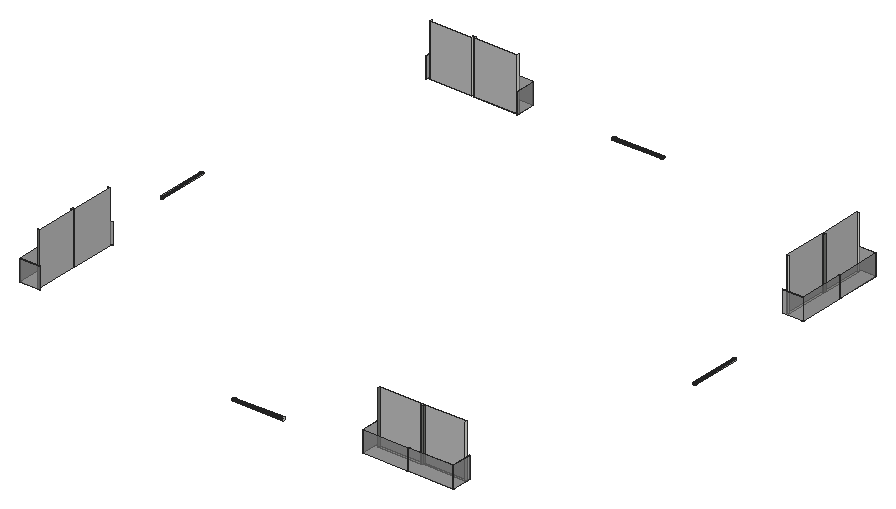
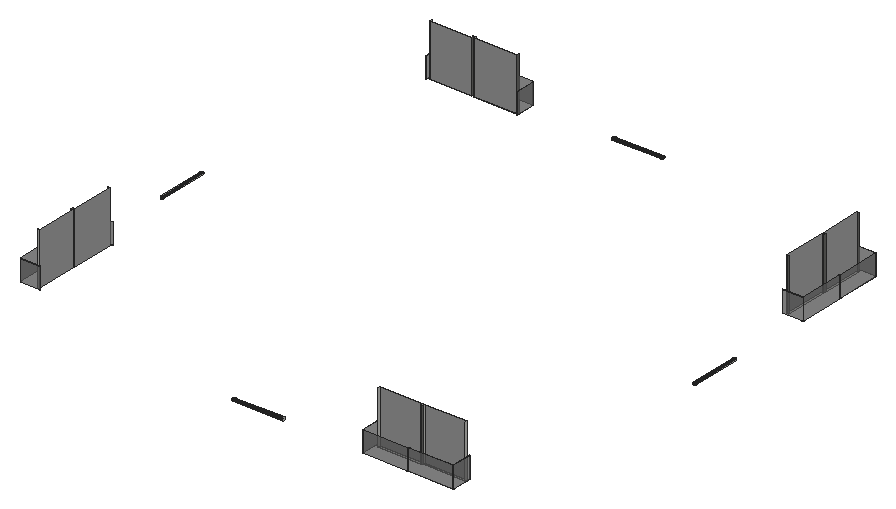
# SketchUp Ruby script. Lengths in inches.
U = 1.inch
M = Sketchup.active_model
def pt(a) = Geom::Point3d.new(a.map { |v| v * U })
def face(e, loops, mat)
  f = e.add_face(loops[0].map { |a| pt(a) })
  loops[1..].each { |l| e.add_face(l.map { |a| pt(a) }).erase! }
  f.material = f.back_material = mat if mat
  f
end
# faces: each face lists its corners as indices into pts; further lists are holes
def faces(e, pts, list, mat = nil) = list.each { |f| face(e, (f[0].is_a?(Array) ? f : [f]).map { |l| l.map { |i| pts[i] } }, mat) }
# xy, xz, yz: faces in a plane at the given z, y or x. An outline is a flat list of corners, or four numbers for a rectangle; further outlines are holes
def ring(l) = l.size == 4 ? [[l[0], l[1]], [l[2], l[1]], [l[2], l[3]], [l[0], l[3]]] : l.each_slice(2).to_a
def flat(e, list, mat, &to3) = list.each { |f| face(e, (f[0].is_a?(Array) ? f : [f]).map { |l| ring(l).map { |u, v| to3.(u, v) } }, mat) }
def xy(e, z, list, mat = nil) = flat(e, list, mat) { |x, y| [x, y, z] }
def xz(e, y, list, mat = nil) = flat(e, list, mat) { |x, z| [x, y, z] }
def yz(e, x, list, mat = nil) = flat(e, list, mat) { |y, z| [x, y, z] }
def lines(e, pts, list) = list.each { |a, b| e.add_line(pt(pts[a]), pt(pts[b])) }
# prism: a flat outline (further loops are holes) pulled along v
def prism(e, loops, v, mat = nil)
  f = face(e, loops, mat); d = Geom::Vector3d.new(v.map { |x| x * U })
  f.pushpull(f.normal.samedirection?(d) ? d.length : -d.length)
end
def box(e, o, s, mat = nil) = prism(e, [[o, [o[0] + s[0], o[1], o[2]], [o[0] + s[0], o[1] + s[1], o[2]], [o[0], o[1] + s[1], o[2]]]], [0, 0, s[2]], mat)
def at(x, y, z, deg = 0) = Geom::Transformation.translation(pt([x, y, z])) * Geom::Transformation.rotation(ORIGIN, Z_AXIS, deg.degrees)
def axes(o, x, y, z) = Geom::Transformation.new([*x, 0, *y, 0, *z, 0, *pt(o).to_a, 1])
def part(name) = M.definitions.add(name)
# library, detail: a bought-in or finely detailed component or shape, given as its bounding box
def library(name, o, s) = part(name).tap { |d| box(d.entities, o, s) }
def detail(e, o, s) = box(e.add_group.entities, o, s)
def put(e, d, t, mat = nil) = e.add_instance(d, t).tap { |i| i.material = mat if mat }
def group(e, t, mat = nil) = e.add_group.tap { |g| g.transformation = t; g.material = mat if mat }.entities
root = M.entities
M.materials.add("[Metal Seamed]").color = [118, 119, 115]
M.materials.add("[Mirror 01]").color = [185, 185, 185]
M.materials.add("[Translucent Glass Tinted]").color = [8, 201, 241]
M.materials["[Translucent Glass Tinted]"].alpha = 0.48
M.materials.add("[Translucent_Glass_Gray]").color = [128, 128, 128]
M.materials["[Translucent_Glass_Gray]"].alpha = 0.5
c1 = part("gler")
box(c1.entities,[0,-0.71,0],[0.37,57.8,41.34],"[Translucent_Glass_Gray]")
xy(root,1219.11,[[1161.2,84.8125,1285.04,90.8125],[1291.04,84.8125,1408.89,90.8125],[120,175.92,126,293.77],[120,299.77,126,423.61],[1494,1126.01,1500,1249.86],
  [1494,1255.86,1500,1373.7],[211.11,1458.8125,328.96,1464.8125],[334.96,1458.8125,458.8,1464.8125]])
xz(root,84.8125,[[1285.04,1219.11,1291.04,1367.61]],"[Metal Seamed]")
xz(root,90.8125,[[1161.2,1219.11,1285.04,1367.61],[1291.04,1219.11,1408.89,1367.61]],"[Mirror 01]")
xz(root,175.92,[[120,1219.11,126,1367.61]],"[Metal Seamed]")
xz(root,293.77,[[120,1219.11,126,1367.61]],"[Metal Seamed]")
xz(root,299.77,[[120,1219.11,126,1367.61]],"[Metal Seamed]")
xz(root,423.61,[[120,1219.11,126,1367.61]],"[Metal Seamed]")
xz(root,662.8,[[83.53,1218.02,84.48,1218.14,85.37,1218.51,86.13,1219.1,86.72,1219.86,87.09,1220.75,87.21,1221.7,87.09,1222.66,86.72,1223.55,86.13,1224.3125,85.37,1224.9,84.48,1225.27,83.53,1225.39,82.57,1225.27,81.68,1224.9,80.92,1224.3125,80.33,1223.55,79.97,1222.66,79.84,1221.7,79.97,1220.75,80.33,1219.86,80.92,1219.1,81.68,1218.51,82.57,1218.14]])
xz(root,886.83,[[1536.47,1218.02,1535.52,1218.14,1534.63,1218.51,1533.87,1219.1,1533.28,1219.86,1532.91,1220.75,1532.79,1221.7,1532.91,1222.66,1533.28,1223.55,1533.87,1224.3125,1534.63,1224.9,1535.52,1225.27,1536.47,1225.39,1537.43,1225.27,1538.32,1224.9,1539.08,1224.3125,1539.67,1223.55,1540.03,1222.66,1540.16,1221.7,1540.03,1220.75,1539.67,1219.86,1539.08,1219.1,1538.32,1218.51,1537.43,1218.14]])
xz(root,1126.01,[[1494,1219.11,1500,1367.61]])
xz(root,1249.86,[[1494,1219.11,1500,1367.61]])
xz(root,1255.86,[[1494,1219.11,1500,1367.61]])
xz(root,1373.7,[[1494,1219.11,1500,1367.61]])
xz(root,1458.8125,[[211.11,1219.11,328.96,1367.61],[334.96,1219.11,458.8,1367.61]],"[Mirror 01]")
xz(root,1464.8125,[[328.96,1219.11,334.96,1367.61]],"[Metal Seamed]")
yz(root,120,[[293.77,1219.11,299.77,1367.61]],"[Metal Seamed]")
yz(root,126,[[175.92,1219.11,293.77,1367.61],[299.77,1219.11,423.61,1367.61]],"[Mirror 01]")
yz(root,211.11,[[1458.8125,1219.11,1464.8125,1367.61]])
yz(root,328.96,[[1458.8125,1219.11,1464.8125,1367.61]])
yz(root,334.96,[[1458.8125,1219.11,1464.8125,1367.61]])
yz(root,458.8,[[1458.8125,1219.11,1464.8125,1367.61]])
yz(root,697.99,[[1501.28,1218.02,1500.33,1218.14,1499.44,1218.51,1498.68,1219.1,1498.09,1219.86,1497.72,1220.75,1497.6,1221.7,1497.72,1222.66,1498.09,1223.55,1498.68,1224.3125,1499.44,1224.9,1500.33,1225.27,1501.28,1225.39,1502.24,1225.27,1503.13,1224.9,1503.89,1224.3125,1504.48,1223.55,1504.85,1222.66,1504.97,1221.7,1504.85,1220.75,1504.48,1219.86,1503.89,1219.1,1503.13,1218.51,1502.24,1218.14]])
yz(root,922.01,[[48.34,1218.02,49.29,1218.14,50.18,1218.51,50.95,1219.1,51.53,1219.86,51.9,1220.75,52.03,1221.7,51.9,1222.66,51.53,1223.55,50.95,1224.3125,50.18,1224.9,49.29,1225.27,48.34,1225.39,47.38,1225.27,46.5,1224.9,45.73,1224.3125,45.15,1223.55,44.78,1222.66,44.65,1221.7,44.78,1220.75,45.15,1219.86,45.73,1219.1,46.5,1218.51,47.38,1218.14]])
yz(root,1161.2,[[84.8125,1219.11,90.8125,1367.61]],"[Metal Seamed]")
yz(root,1285.04,[[84.8125,1219.11,90.8125,1367.61]])
yz(root,1291.04,[[84.8125,1219.11,90.8125,1367.61]],"[Metal Seamed]")
yz(root,1408.89,[[84.8125,1219.11,90.8125,1367.61]])
yz(root,1494,[[1126.01,1219.11,1249.86,1367.61],[1255.86,1219.11,1373.7,1367.61]],"[Mirror 01]")
yz(root,1500,[[1249.86,1219.11,1255.86,1367.61]],"[Metal Seamed]")
p = [[922.01,48.34,1218.02],[922.01,47.38,1218.14],[778.64,47.38,1218.14],[778.64,48.34,1218.02],[922.01,49.29,1218.14],[778.64,49.29,1218.14],
  [83.53,662.8,1218.02],[82.57,662.8,1218.14],[82.57,806.17,1218.14],[83.53,806.17,1218.02],[84.48,662.8,1218.14],[84.48,806.17,1218.14],
  [1535.52,886.83,1218.14],[1536.47,886.83,1218.02],[1536.47,743.45,1218.02],[1535.52,743.45,1218.14],[1537.43,886.83,1218.14],[1537.43,743.45,1218.14],
  [697.99,1500.33,1218.14],[697.99,1501.28,1218.02],[841.36,1501.28,1218.02],[841.36,1500.33,1218.14],[697.99,1502.24,1218.14],[841.36,1502.24,1218.14],
  [922.01,46.5,1218.51],[778.64,46.5,1218.51],[922.01,50.18,1218.51],[778.64,50.18,1218.51],[81.68,662.8,1218.51],[81.68,806.17,1218.51],
  [85.37,662.8,1218.51],[85.37,806.17,1218.51],[1534.63,886.83,1218.51],[1534.63,743.45,1218.51],[1538.32,886.83,1218.51],[1538.32,743.45,1218.51],
  [697.99,1499.44,1218.51],[841.36,1499.44,1218.51],[697.99,1503.13,1218.51],[841.36,1503.13,1218.51],[922.01,45.73,1219.1],[778.64,45.73,1219.1],
  [922.01,50.95,1219.1],[778.64,50.95,1219.1],[80.92,662.8,1219.1],[80.92,806.17,1219.1],[86.13,662.8,1219.1],[86.13,806.17,1219.1],
  [1533.87,886.83,1219.1],[1533.87,743.45,1219.1],[1539.08,886.83,1219.1],[1539.08,743.45,1219.1],[697.99,1498.68,1219.1],[841.36,1498.68,1219.1],
  [697.99,1503.89,1219.1],[841.36,1503.89,1219.1],[922.01,45.15,1219.86],[778.64,45.15,1219.86],[922.01,51.53,1219.86],[778.64,51.53,1219.86],
  [80.33,662.8,1219.86],[80.33,806.17,1219.86],[86.72,662.8,1219.86],[86.72,806.17,1219.86],[1533.28,886.83,1219.86],[1533.28,743.45,1219.86],
  [1539.67,886.83,1219.86],[1539.67,743.45,1219.86],[697.99,1498.09,1219.86],[841.36,1498.09,1219.86],[697.99,1504.48,1219.86],[841.36,1504.48,1219.86],
  [922.01,44.78,1220.75],[778.64,44.78,1220.75],[922.01,51.9,1220.75],[778.64,51.9,1220.75],[79.97,662.8,1220.75],[79.97,806.17,1220.75],
  [87.09,662.8,1220.75],[87.09,806.17,1220.75],[1532.91,886.83,1220.75],[1532.91,743.45,1220.75],[1540.03,886.83,1220.75],[1540.03,743.45,1220.75],
  [697.99,1497.72,1220.75],[841.36,1497.72,1220.75],[697.99,1504.85,1220.75],[841.36,1504.85,1220.75],[922.01,44.65,1221.7],[778.64,44.65,1221.7],
  [922.01,52.03,1221.7],[778.64,52.03,1221.7],[79.84,662.8,1221.7],[79.84,806.17,1221.7],[87.21,662.8,1221.7],[87.21,806.17,1221.7],
  [1532.79,886.83,1221.7],[1532.79,743.45,1221.7],[1540.16,886.83,1221.7],[1540.16,743.45,1221.7],[697.99,1497.6,1221.7],[841.36,1497.6,1221.7],
  [697.99,1504.97,1221.7],[841.36,1504.97,1221.7],[922.01,44.78,1222.66],[778.64,44.78,1222.66],[922.01,51.9,1222.66],[778.64,51.9,1222.66],
  [79.97,662.8,1222.66],[79.97,806.17,1222.66],[87.09,662.8,1222.66],[87.09,806.17,1222.66],[1532.91,886.83,1222.66],[1532.91,743.45,1222.66],
  [1540.03,886.83,1222.66],[1540.03,743.45,1222.66],[697.99,1497.72,1222.66],[841.36,1497.72,1222.66],[697.99,1504.85,1222.66],[841.36,1504.85,1222.66],
  [922.01,45.15,1223.55],[778.64,45.15,1223.55],[922.01,51.53,1223.55],[778.64,51.53,1223.55],[80.33,662.8,1223.55],[80.33,806.17,1223.55],
  [86.72,662.8,1223.55],[86.72,806.17,1223.55],[1533.28,886.83,1223.55],[1533.28,743.45,1223.55],[1539.67,886.83,1223.55],[1539.67,743.45,1223.55],
  [697.99,1498.09,1223.55],[841.36,1498.09,1223.55],[697.99,1504.48,1223.55],[841.36,1504.48,1223.55],[922.01,45.73,1224.3125],[778.64,45.73,1224.3125],
  [922.01,50.95,1224.3125],[778.64,50.95,1224.3125],[80.92,662.8,1224.3125],[80.92,806.17,1224.3125],[86.13,662.8,1224.3125],[86.13,806.17,1224.3125],
  [1533.87,886.83,1224.3125],[1533.87,743.45,1224.3125],[1539.08,886.83,1224.3125],[1539.08,743.45,1224.3125],[697.99,1498.68,1224.3125],[841.36,1498.68,1224.3125],
  [697.99,1503.89,1224.3125],[841.36,1503.89,1224.3125],[922.01,46.5,1224.9],[778.64,46.5,1224.9],[922.01,50.18,1224.9],[778.64,50.18,1224.9],
  [81.68,662.8,1224.9],[81.68,806.17,1224.9],[85.37,662.8,1224.9],[85.37,806.17,1224.9],[1534.63,886.83,1224.9],[1534.63,743.45,1224.9],
  [1538.32,886.83,1224.9],[1538.32,743.45,1224.9],[697.99,1499.44,1224.9],[841.36,1499.44,1224.9],[697.99,1503.13,1224.9],[841.36,1503.13,1224.9],
  [922.01,48.34,1221.7],[778.64,48.34,1221.7],[697.99,1501.28,1221.7],[841.36,1501.28,1221.7],[1536.47,886.83,1221.7],[1536.47,743.45,1221.7],
  [83.53,662.8,1221.7],[83.53,806.17,1221.7]]
faces(root,p,[[0,1,2,3],[4,0,3,5],[6,7,8,9],[10,6,9,11],[12,13,14,15],[13,16,17,14],[18,19,20,21],[19,22,23,20],
  [1,24,25,2],[26,4,5,27],[7,28,29,8],[30,10,11,31],[32,12,15,33],[16,34,35,17],[36,18,21,37],[22,38,39,23],
  [24,40,41,25],[42,26,27,43],[28,44,45,29],[46,30,31,47],[48,32,33,49],[34,50,51,35],[52,36,37,53],[38,54,55,39],
  [40,56,57,41],[58,42,43,59],[44,60,61,45],[62,46,47,63],[64,48,49,65],[50,66,67,51],[68,52,53,69],[54,70,71,55],
  [56,72,73,57],[74,58,59,75],[60,76,77,61],[78,62,63,79],[80,64,65,81],[66,82,83,67],[84,68,69,85],[70,86,87,71],
  [72,88,89,73],[90,74,75,91],[76,92,93,77],[94,78,79,95],[96,80,81,97],[82,98,99,83],[100,84,85,101],[86,102,103,87],
  [88,104,105,89],[106,90,91,107],[92,108,109,93],[110,94,95,111],[112,96,97,113],[98,114,115,99],[116,100,101,117],[102,118,119,103],
  [104,120,121,105],[122,106,107,123],[108,124,125,109],[126,110,111,127],[128,112,113,129],[114,130,131,115],[132,116,117,133],[118,134,135,119],
  [120,136,137,121],[138,122,123,139],[124,140,141,125],[142,126,127,143],[144,128,129,145],[130,146,147,131],[148,132,133,149],[134,150,151,135],
  [136,152,153,137],[154,138,139,155],[140,156,157,141],[158,142,143,159],[160,144,145,161],[146,162,163,147],[164,148,149,165],[150,166,167,151]])
lines(root,p,[[168,169],[170,171],[172,173],[174,175]])
put(root,c1,axes([1414.89,96.58,1218.03],[-2.19843,0,0],[0,-1,0],[0,0,1.5]),"[Translucent Glass Tinted]")
put(root,c1,axes([208.38,1511,1218.03],[0,-1,0],[2.19843,0,0],[0,0,1.5]),"[Translucent Glass Tinted]")
put(root,c1,axes([337.35,1511,1218.03],[0,-1,0],[2.19843,0,0],[0,0,1.5]),"[Translucent Glass Tinted]")
put(root,c1,axes([1155.97,96.58,1218.03],[-2.19843,0,0],[0,-1,0],[0,0,1.5]),"[Translucent Glass Tinted]")
put(root,c1,axes([1546.19,1247.46,1218.03],[-1,0,0],[0,-2.19843,0],[0,0,1.5]),"[Translucent Glass Tinted]")
put(root,c1,axes([1546.19,1376.43,1218.03],[-1,0,0],[0,-2.19843,0],[0,0,1.5]),"[Translucent Glass Tinted]")
put(root,c1,axes([1488.23,1120.78,1218.03],[0,-2.19843,0],[1,0,0],[0,0,1.5]),"[Translucent Glass Tinted]")
put(root,c1,axes([131.77,169.92,1218.03],[0,2.19843,0],[-1,0,0],[0,0,1.5]),"[Translucent Glass Tinted]")
put(root,c1,axes([1488.23,1379.7,1218.03],[0,-2.19843,0],[1,0,0],[0,0,1.5]),"[Translucent Glass Tinted]")
put(root,c1,axes([464.03,1453.04,1218.03],[2.19843,0,0],[0,1,0],[0,0,1.5]),"[Translucent Glass Tinted]")
put(root,c1,axes([205.11,1453.04,1218.03],[2.19843,0,0],[0,1,0],[0,0,1.5]),"[Translucent Glass Tinted]")
put(root,c1,axes([73.81,173.19,1218.03],[1,0,0],[0,2.19843,0],[0,0,1.5]),"[Translucent Glass Tinted]")
put(root,c1,axes([73.81,302.16,1218.03],[1,0,0],[0,2.19843,0],[0,0,1.5]),"[Translucent Glass Tinted]")
put(root,c1,axes([1411.62,38.625,1218.03],[0,1,0],[-2.19843,0,0],[0,0,1.5]),"[Translucent Glass Tinted]")
put(root,c1,axes([1282.65,38.625,1218.03],[0,1,0],[-2.19843,0,0],[0,0,1.5]),"[Translucent Glass Tinted]")
put(root,c1,axes([131.77,428.84,1218.03],[0,2.19843,0],[-1,0,0],[0,0,1.5]),"[Translucent Glass Tinted]")
